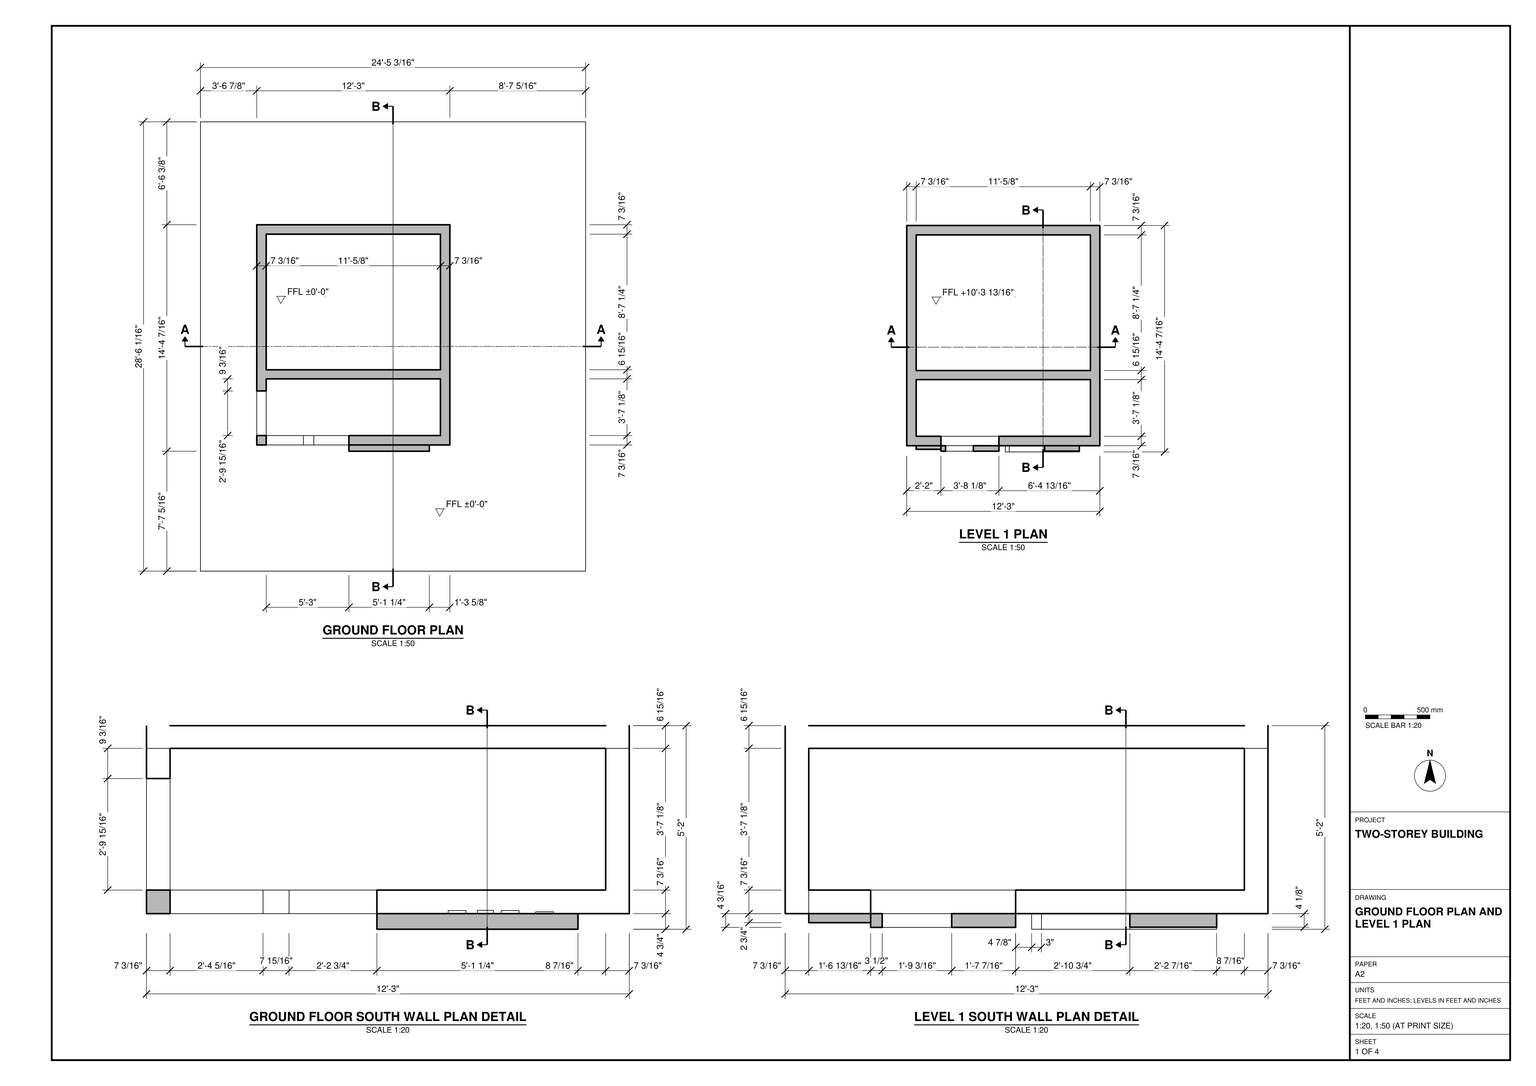
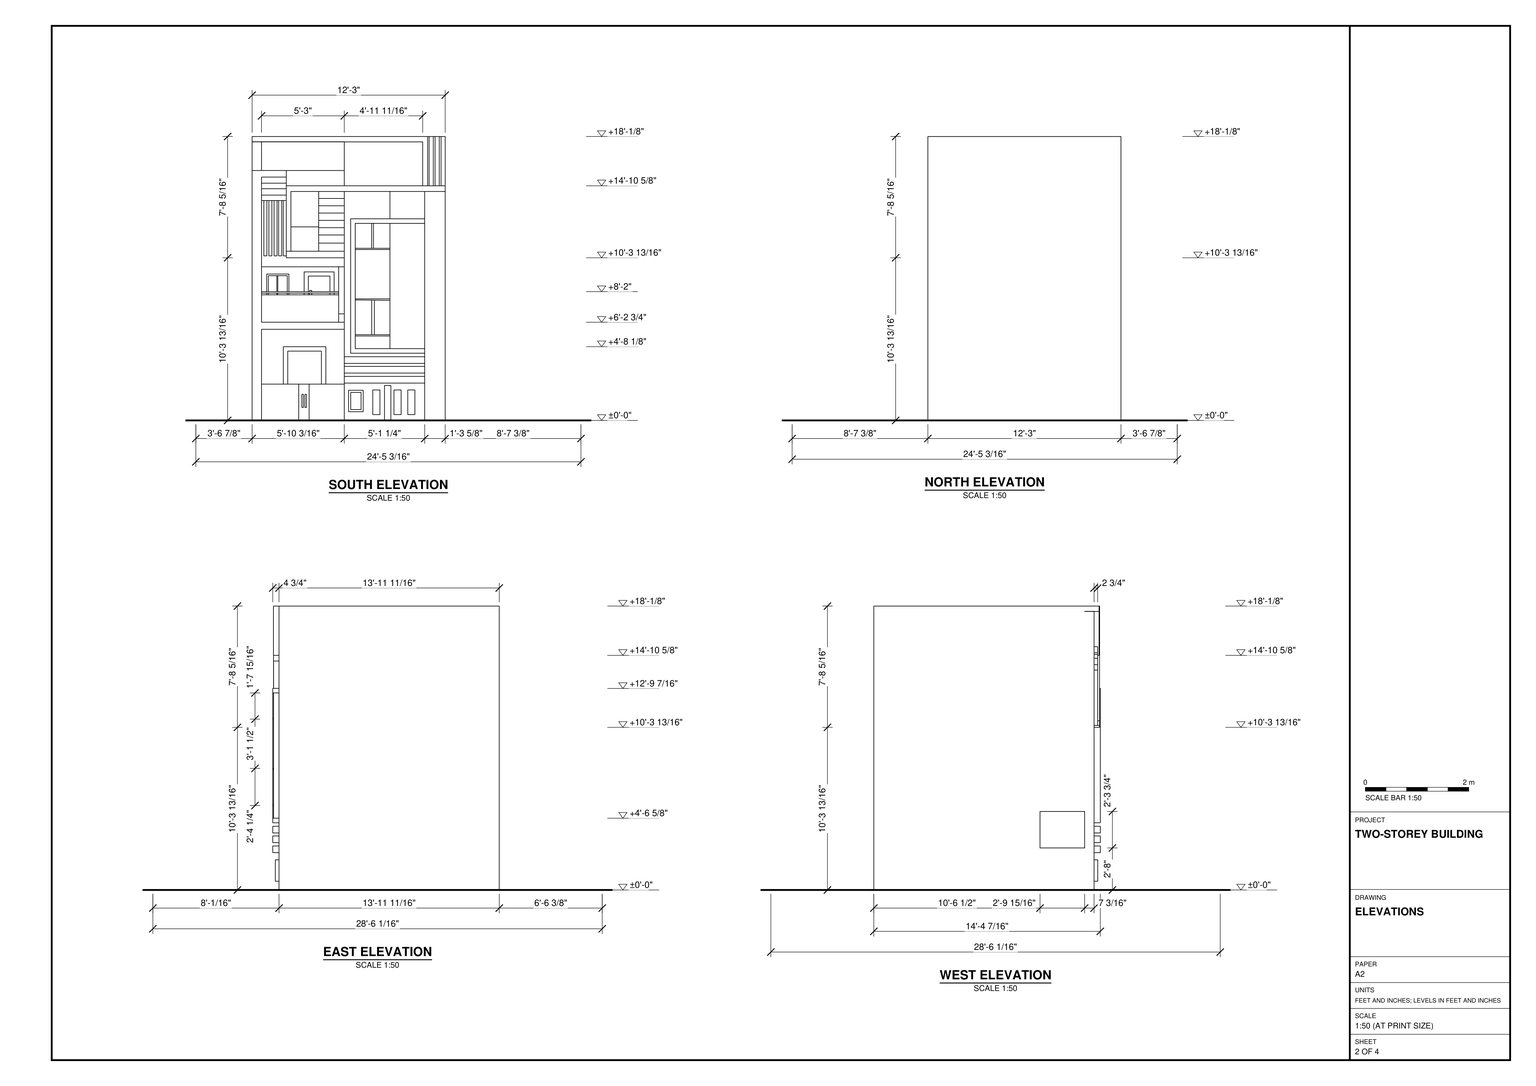
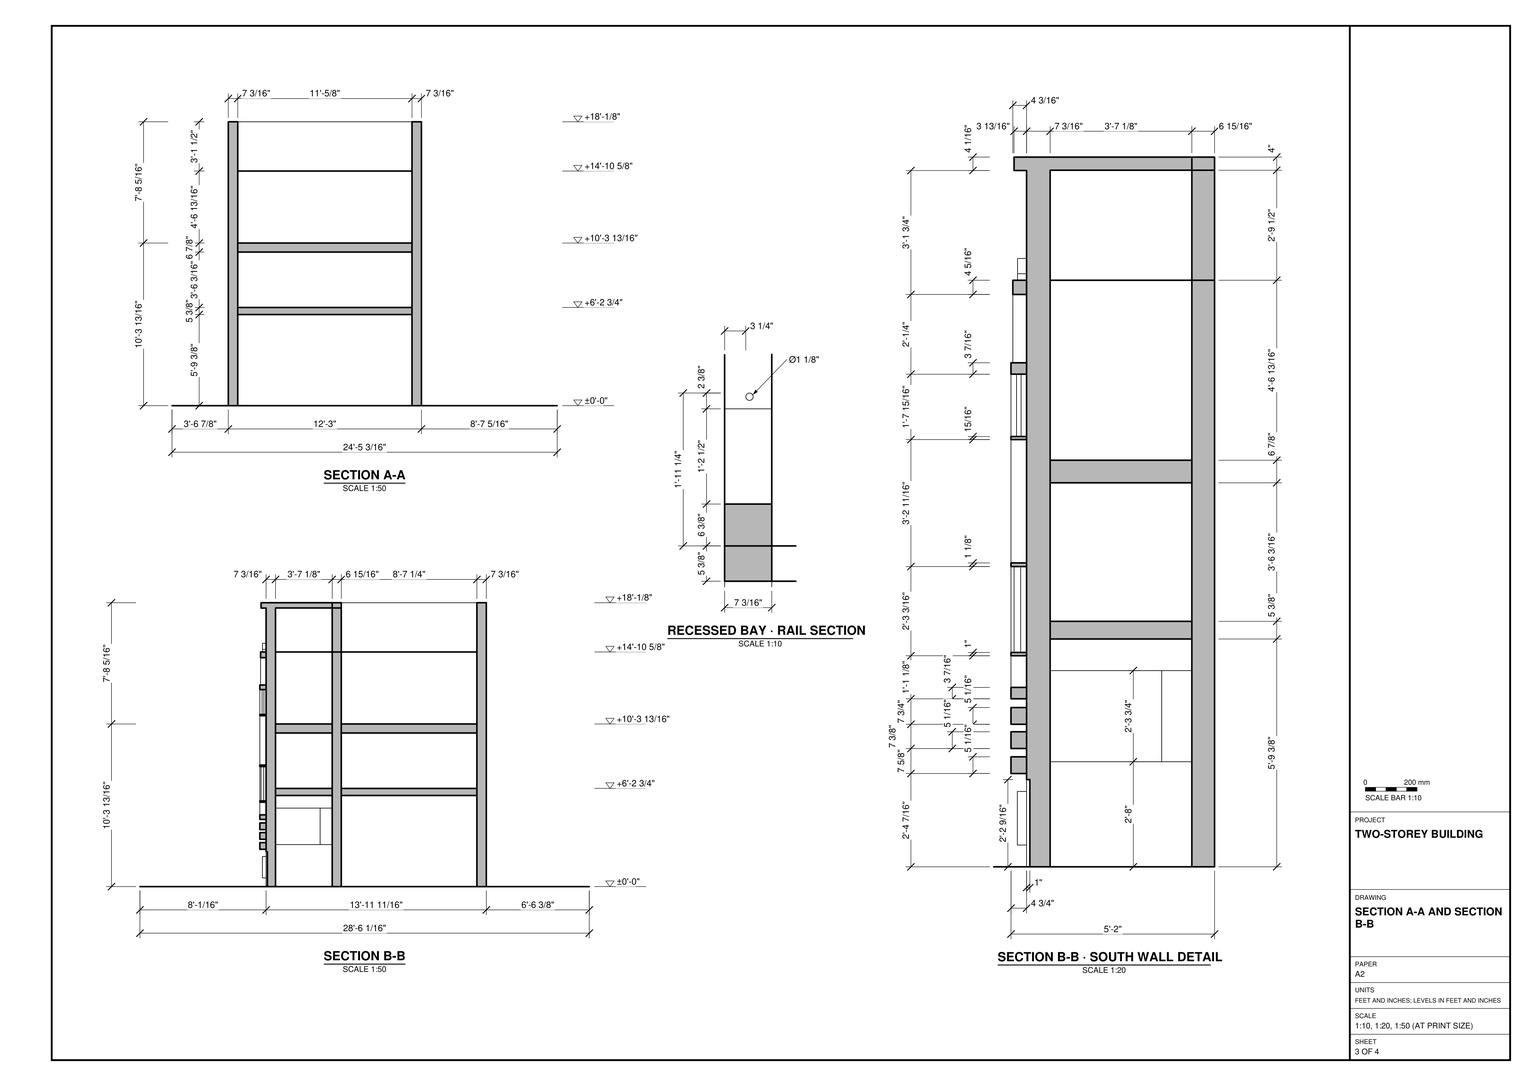
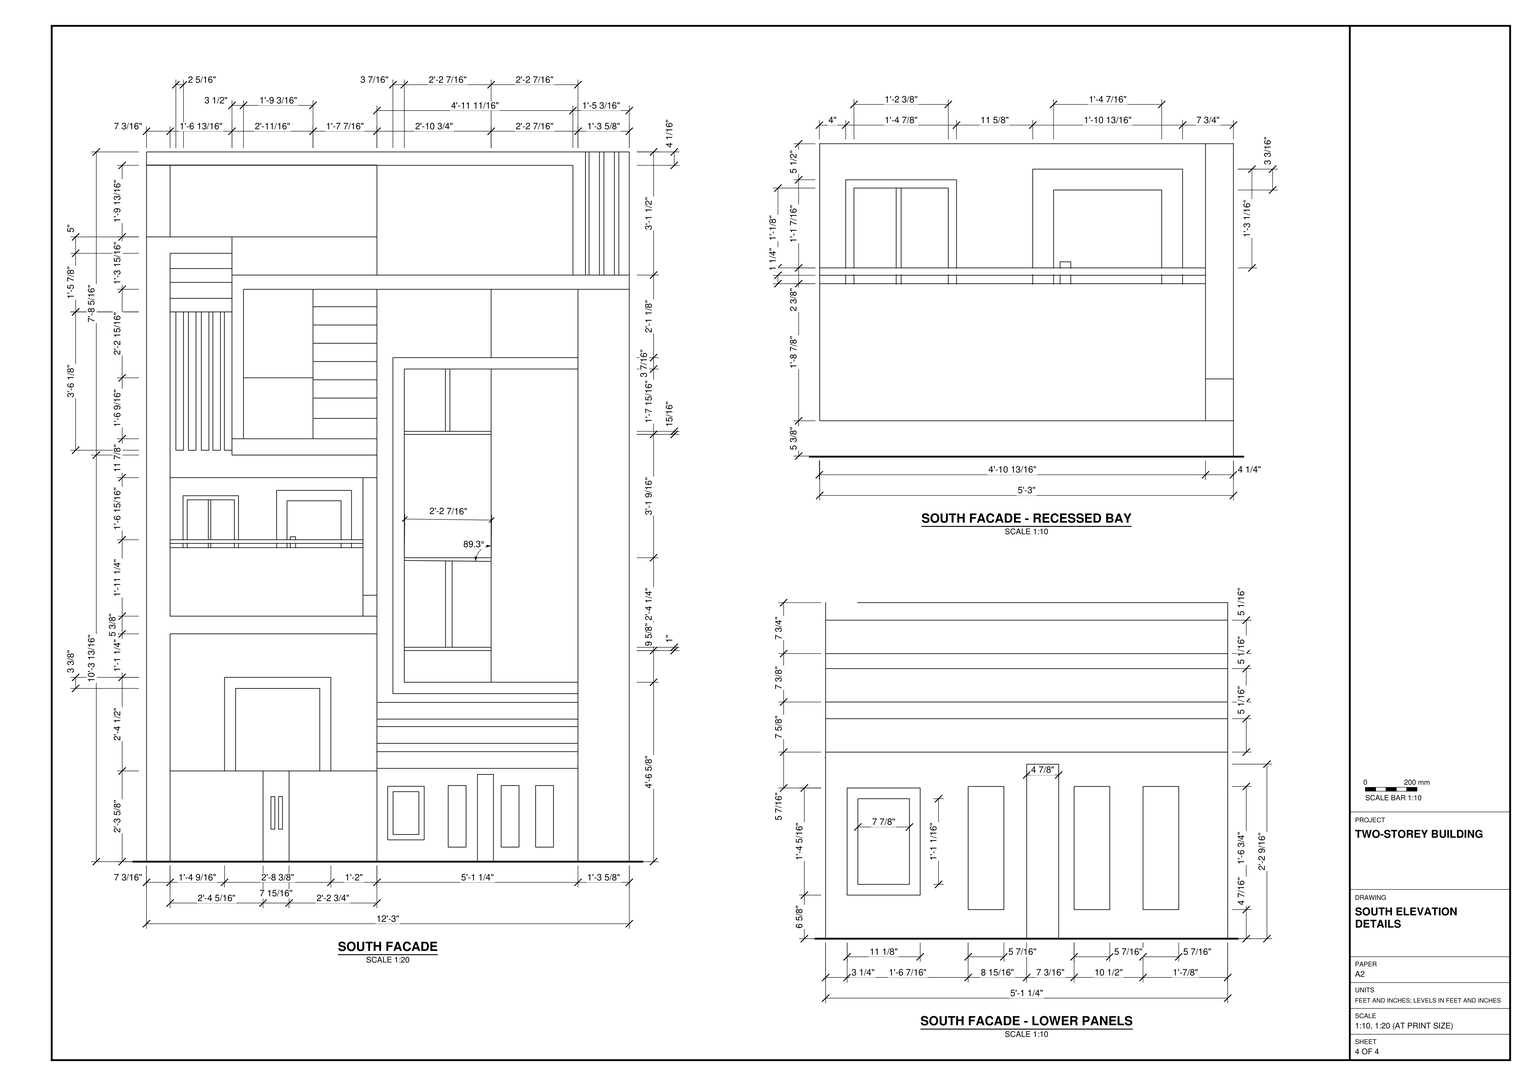
Use task_files/diagram_01.pdf to build the model in SketchUp. Work in feet and inches. Include the rectangular ground plane: the overall model measures 24'-5 3/16" east to west, 28'-6 1/16" north to south and 18'-1/8" high. Set the ground floor at ±0'-0" and Level 1 at +10'-3 13/16". Position the building on the ground plane using the offsets in the ground floor plan rather than centring it.

Build the 12'-3" wide shell with 7 3/16" exterior walls. Set the transverse wall behind the shallow south bay at the thickness shown, leaving the larger space to the north. Use sections A-A and B-B to place the slabs, the intermediate horizontal element below Level 1 and the roof cap over the south bay. Keep the north and east faces plain and include the low opening near the south end of the west wall.

Use the enlarged south wall plans and section to give the frontage depth. Include the entrance panels, recessed bay with its rail, vertical slats, tall framed panel assembly and projecting horizontal bands. Keep shell elements such as walls, slabs and roof, and each furniture or joinery piece, in separate groups or components; use components for repeated parts. Any decor or loose items shown may be suitable library components. Save one SketchUp model as output_files/two_storey_building_with_a_recessed_south_bay.skp.

# SketchUp Ruby script. Lengths in inches.
U = 1.inch
M = Sketchup.active_model
def pt(a) = Geom::Point3d.new(a.map { |v| v * U })
def face(e, loops, mat)
  f = e.add_face(loops[0].map { |a| pt(a) })
  loops[1..].each { |l| e.add_face(l.map { |a| pt(a) }).erase! }
  f.material = f.back_material = mat if mat
  f
end
# faces: each face lists its corners as indices into pts; further lists are holes
def faces(e, pts, list, mat = nil) = list.each { |f| face(e, (f[0].is_a?(Array) ? f : [f]).map { |l| l.map { |i| pts[i] } }, mat) }
# xy, xz, yz: faces in a plane at the given z, y or x. An outline is a flat list of corners, or four numbers for a rectangle; further outlines are holes
def ring(l) = l.size == 4 ? [[l[0], l[1]], [l[2], l[1]], [l[2], l[3]], [l[0], l[3]]] : l.each_slice(2).to_a
def flat(e, list, mat, &to3) = list.each { |f| face(e, (f[0].is_a?(Array) ? f : [f]).map { |l| ring(l).map { |u, v| to3.(u, v) } }, mat) }
def xy(e, z, list, mat = nil) = flat(e, list, mat) { |x, y| [x, y, z] }
def xz(e, y, list, mat = nil) = flat(e, list, mat) { |x, z| [x, y, z] }
def yz(e, x, list, mat = nil) = flat(e, list, mat) { |y, z| [x, y, z] }
def lines(e, pts, list) = list.each { |a, b| e.add_line(pt(pts[a]), pt(pts[b])) }
# prism: a flat outline (further loops are holes) pulled along v
def prism(e, loops, v, mat = nil)
  f = face(e, loops, mat); d = Geom::Vector3d.new(v.map { |x| x * U })
  f.pushpull(f.normal.samedirection?(d) ? d.length : -d.length)
end
def box(e, o, s, mat = nil) = prism(e, [[o, [o[0] + s[0], o[1], o[2]], [o[0] + s[0], o[1] + s[1], o[2]], [o[0], o[1] + s[1], o[2]]]], [0, 0, s[2]], mat)
def at(x, y, z, deg = 0) = Geom::Transformation.translation(pt([x, y, z])) * Geom::Transformation.rotation(ORIGIN, Z_AXIS, deg.degrees)
def axes(o, x, y, z) = Geom::Transformation.new([*x, 0, *y, 0, *z, 0, *pt(o).to_a, 1])
def part(name) = M.definitions.add(name)
# library, detail: a bought-in or finely detailed component or shape, given as its bounding box
def library(name, o, s) = part(name).tap { |d| box(d.entities, o, s) }
def detail(e, o, s) = box(e.add_group.entities, o, s)
def put(e, d, t, mat = nil) = e.add_instance(d, t).tap { |i| i.material = mat if mat }
def group(e, t, mat = nil) = e.add_group.tap { |g| g.transformation = t; g.material = mat if mat }.entities
root = M.entities
M.materials.add("[Aluminum]").color = [179, 179, 179]
M.materials.add("[Asphalt New]").color = [67, 60, 62]
M.materials.add("[Blinds Cellular White]").color = [217, 211, 213]
M.materials.add("[Blinds Cloth Horizontal]").color = [192, 163, 85]
M.materials.add("[Blinds Weave]").color = [141, 91, 25]
M.materials.add("[Color A02]").color = [255, 153, 153]
M.materials.add("[Color A08]").color = [102, 0, 0]
M.materials.add("[Formica Laminate Dark]").color = [50, 53, 60]
M.materials.add("[Formica Laminate Light]").color = [213, 189, 164]
M.materials.add("[Marble Carrara Gold Floor Tile]").color = [225, 223, 217]
M.materials.add("[Polished Concrete Old]").color = [229, 229, 229]
M.materials.add("[Quartz Light Brown]").color = [199, 184, 152]
M.materials.add("[Terrazzo Tile Light]").color = [219, 217, 210]
M.materials.add("[Translucent Glass Blue]").color = [100, 149, 237]
M.materials["[Translucent Glass Blue]"].alpha = 0.5
M.materials.add("[Wood Bamboo]").color = [177, 105, 43]
M.materials.add("[Wood Cherry Original]").color = [152, 86, 42]
M.materials.add("[Wood Floor Dark]").color = [153, 94, 42]
M.materials.add("[Wood OSB]").color = [240, 195, 122]
M.materials.add("[Wood Veneer 01]").color = [120, 70, 37]
M.materials.add("[Wood Veneer 02]").color = [190, 128, 91]
xy(root,0,[[[0,0,293.1875,342.0625],[42.85,96.04,42.85,263.7,189.85,263.7,189.85,96.04,148.5,96.04,148.5,97.04,143.625,97.04,143.625,96.04]],[42.85,96.04,78.34,103.22],[78.34,96.04,86.26,103.22],[86.26,96.04,143.625,96.04,143.625,97.04,148.5,97.04,148.5,96.04,189.85,96.04,189.85,146.37,182.67,146.37,182.67,103.22,86.26,103.22],[42.85,103.22,50.03,146.37],
  [50.03,103.22,182.67,146.37],[[42.85,146.37,189.85,263.7],[50.03,153.28,182.67,256.52]],[50.03,153.28,182.67,256.52]])
xy(root,4.43,[[134.72,96.04,140.15,96.98],[150.84,96.04,156.28,96.98],[161.34,96.04,166.78,96.6]])
xy(root,6.63,[[116.29,93.23,127.41,96.04]])
xy(root,8.27,[[117.92,93.23,125.78,96.04]])
xy(root,21.3125,[[117.92,93.23,125.78,96.04]])
xy(root,22.95,[[116.29,93.23,127.41,96.04]])
xy(root,23.18,[[134.72,96.04,140.15,96.98],[150.84,96.04,156.28,96.98],[161.34,96.04,166.78,96.6]])
xy(root,26.5625,[[143.625,96.04,148.5,97.04]])
xy(root,27.62,[[50.03,96.04,78.34,103.22],[78.34,96.04,86.26,103.22],[86.26,96.04,113.01,103.22]],"[Formica Laminate Dark]")
xy(root,28.41,[[113.01,91.29,174.23,96.04]],"[Color A02]")
xy(root,32,[[42.85,103.22,50.03,137.18]],"[Quartz Light Brown]")
xy(root,33.5,[[113.01,91.29,174.23,96.04]],"[Color A02]")
xy(root,36.03,[[113.01,91.29,174.23,96.04]],"[Color A02]")
xy(root,41.12,[[113.01,91.29,174.23,96.04]],"[Color A02]")
xy(root,43.41,[[113.01,91.29,174.23,96.04]],"[Color A02]")
xy(root,48.5,[[113.01,91.29,174.23,96.04]],"[Color A02]")
xy(root,51.17,[[117.88,91.29,120.88,96.04],[120.88,91.29,174.23,96.04]])
xy(root,54.64,[[147.79,91.29,174.23,91.91],[147.79,91.91,174.23,96.04]])
xy(root,54.64,[[121.35,91.29,147.79,96.04]],"[Wood Veneer 01]")
xy(root,59.75,[[42.85,103.22,50.03,137.18]])
xy(root,64.28,[[121.35,91.29,147.79,96.04]],"[Wood Veneer 01]")
xy(root,65.28,[[[121.35,91.29,147.79,96.04],[134.91,92.23,134.65,92.26,134.41,92.36,134.2,92.52,134.05,92.73,133.95,92.97,133.91,93.23,133.95,93.49,134.05,93.73,134.2,93.9375,134.41,94.1,134.65,94.2,134.91,94.23,135.17,94.2,135.41,94.1,135.62,93.9375,135.78,93.73,135.88,93.49,135.91,93.23,135.88,92.97,135.78,92.73,135.62,92.52,135.41,92.36,135.17,92.26]],[134.91,92.23,134.65,92.26,134.41,92.36,134.2,92.52,134.05,92.73,133.95,92.97,133.91,93.23,133.95,93.49,134.05,93.73,134.2,93.9375,134.41,94.1,134.65,94.2,134.91,94.23,135.17,94.2,135.41,94.1,135.62,93.9375,135.78,93.73,135.88,93.49,135.91,93.23,135.88,92.97,135.78,92.73,135.62,92.52,135.41,92.36,135.17,92.26]])
xy(root,69.375,[[50.03,96.04,113.01,103.22],[50.03,103.22,182.67,146.37],[50.03,153.28,182.67,256.52]])
xy(root,74.75,[[50.03,96.04,113.01,103.22],[50.03,103.22,182.67,146.37],[50.03,153.28,182.67,256.52]])
xy(root,81.125,[[108.76,96.04,113.01,103.22]])
xy(root,91.5625,[[134.91,92.23,135.17,92.26,135.41,92.36,135.62,92.52,135.78,92.73,135.88,92.97,135.91,93.23,135.88,93.49,135.78,93.73,135.62,93.9375,135.41,94.1,135.17,94.2,134.91,94.23,134.65,94.2,134.41,94.1,134.2,93.9375,134.05,93.73,133.95,93.49,133.91,93.23,133.95,92.97,134.05,92.73,134.2,92.52,134.41,92.36,134.65,92.26]])
xy(root,92.55,[[121.35,91.29,147.79,96.04]],"[Wood Veneer 01]")
xy(root,95.625,[[50.03,96.04,108.76,103.22]],"[Translucent Glass Blue]")
xy(root,116.9375,[[50.03,96.04,108.76,103.22],[108.76,96.04,113.01,103.22],[50.03,103.22,182.67,146.37],[50.03,153.28,182.67,256.52]])
xy(root,123.8125,[[68.87,96.04,113.01,103.22],[50.03,103.22,182.67,146.37],[50.03,153.28,182.67,256.52]])
xy(root,123.8125,[[68.87,91.85,113.01,96.04]],"[Color A08]")
xy(root,125.28,[[51.8,93.29,54.11,96.04],[55.61,93.29,57.92,96.04],[59.55,93.29,61.86,96.04],[63.05,93.29,65.37,96.04],[66.56,93.29,68.87,96.04]])
xy(root,128.78,[[68.87,91.85,72.38,96.04]])
xy(root,128.78,[[72.38,91.85,93.55,96.04]],"[Color A08]")
xy(root,130.1,[[121.35,91.29,147.79,96.04]],"[Wood Veneer 01]")
xy(root,131.04,[[[121.35,91.29,147.79,96.04],[134.55,92.99,134.37,93.01,134.2,93.08,134.0625,93.19,133.95,93.33,133.88,93.5,133.86,93.68,133.88,93.85,133.95,94.02,134.0625,94.16,134.2,94.27,134.37,94.34,134.55,94.36,134.73,94.34,134.89,94.27,135.03,94.16,135.14,94.02,135.21,93.85,135.24,93.68,135.21,93.5,135.14,93.33,135.03,93.19,134.89,93.08,134.73,93.01]],[134.55,92.99,134.37,93.01,134.2,93.08,134.0625,93.19,133.95,93.33,133.88,93.5,133.86,93.68,133.88,93.85,133.95,94.02,134.0625,94.16,134.2,94.27,134.37,94.34,134.55,94.36,134.73,94.34,134.89,94.27,135.03,94.16,135.14,94.02,135.21,93.85,135.24,93.68,135.21,93.5,135.14,93.33,135.03,93.19,134.89,93.08,134.73,93.01]])
xy(root,147.34,[[68.87,96.04,113.01,103.22]],"[Translucent Glass Blue]")
xy(root,150.02,[[[121.35,91.29,147.79,96.04],[134.55,92.99,134.73,93.01,134.89,93.08,135.03,93.19,135.14,93.33,135.21,93.5,135.24,93.68,135.21,93.85,135.14,94.02,135.03,94.16,134.89,94.27,134.73,94.34,134.55,94.36,134.37,94.34,134.2,94.27,134.0625,94.16,133.95,94.02,133.88,93.85,133.86,93.68,133.88,93.5,133.95,93.33,134.0625,93.19,134.2,93.08,134.37,93.01]],[147.79,91.29,174.23,91.91],[147.79,91.91,174.23,96.04]])
xy(root,153.49,[[117.88,91.29,120.88,96.04],[120.88,91.29,147.79,96.04],[147.79,91.29,174.23,91.91],[147.79,91.91,174.23,96.04]])
xy(root,167.41,[[50.03,93.29,51.8,96.04],[51.8,93.29,54.11,96.04],[54.11,93.29,55.61,96.04],[55.61,93.29,57.92,96.04],[57.92,93.29,59.55,96.04],
  [59.55,93.29,61.86,96.04],[61.86,93.29,63.05,96.04],[63.05,93.29,65.37,96.04],[65.37,93.29,66.56,96.04],[66.56,93.29,68.87,96.04]])
xy(root,171.54,[[50.03,93.29,68.87,96.04]])
xy(root,174.29,[[147.79,91.91,174.23,96.04],[68.87,96.04,113.01,103.22]])
xy(root,174.29,[[72.38,91.85,93.55,96.04],[113.01,91.85,113.01,96.04,147.79,96.04,147.79,91.91,174.23,91.91,174.23,96.04,189.85,96.04,189.85,91.85]],"[Color A08]")
xy(root,176.39,[[50.03,93.29,68.87,96.04]])
xy(root,178.625,[[172.7,92.23,176.51,96.04],[68.87,96.04,113.01,103.22],[50.03,103.22,182.67,146.37],[50.03,146.37,114.88,153.28],[114.88,146.37,182.67,153.28],
  [50.03,153.28,182.67,256.52]])
xy(root,178.625,[[177.6,91.79,180.78,91.85],[182.14,91.79,185.32,91.85],[186.67,91.79,189.85,91.85],[68.87,91.85,177.6,91.85,177.6,96.04,176.51,96.04,176.51,92.23,172.7,92.23,172.7,96.04,68.87,96.04],[177.6,91.85,180.78,96.04],
  [180.78,91.85,182.14,96.04],[182.14,91.85,185.32,96.04],[185.32,91.85,186.67,96.04],[186.67,91.85,189.85,96.04]],"[Color A08]")
xy(root,180.62,[[50.03,93.29,68.87,96.04]])
xy(root,185.26,[[50.03,93.29,68.87,96.04]],"[Wood Cherry Original]")
xy(root,190.25,[[50.03,96.04,68.87,103.22]],"[Color A08]")
xy(root,190.25,[[68.87,96.04,113.01,103.22]],"[Translucent Glass Blue]")
xy(root,212.04,[[113.01,92.23,172.7,96.04],[42.85,96.04,50.03,103.22]])
xy(root,212.04,[[42.85,92.23,50.03,95.84],[50.03,92.23,113.01,96.04],[42.85,95.84,50.03,96.04]],"[Color A08]")
xy(root,212.125,[[42.85,95.84,50.03,103.22],[114.88,146.37,182.67,153.28]])
xy(root,212.125,[[[50.03,103.22,182.67,146.37],[55.6875,107.83,60.6875,139.15],[62.5,107.83,67.5,139.15],[69.5,107.83,74.5,139.15],[76.75,107.83,81.75,139.15],[84.0625,107.83,89.0625,139.15],[91.625,107.83,96.625,139.15],[99.5625,107.83,104.5625,139.15],[106.9375,107.83,111.9375,139.15]]],"[Quartz Light Brown]")
xy(root,216.125,[[[50.03,103.22,182.67,146.37],[55.6875,107.83,60.6875,139.15],[62.5,107.83,67.5,139.15],[69.5,107.83,74.5,139.15],[76.75,107.83,81.75,139.15],[84.0625,107.83,89.0625,139.15],[91.625,107.83,96.625,139.15],[99.5625,107.83,104.5625,139.15],[106.9375,107.83,111.9375,139.15]]],"[Color A08]")
xy(root,216.125,[[177.6,91.79,180.78,96.04],[182.14,91.79,185.32,96.04],[186.67,91.79,189.85,96.04]],"[Polished Concrete Old]")
xy(root,216.125,[[42.85,92.23,176.51,92.23,176.51,96.04,189.85,96.04,189.85,263.7,42.85,263.7,42.85,103.22,50.03,103.22,50.03,256.52,182.67,256.52,182.67,153.28,114.88,153.28,114.88,146.37,182.67,146.37,182.67,103.22,42.85,103.22]],"[Quartz Light Brown]")
xz(root,91.29,[[117.88,51.17,174.23,51.17,174.23,54.64,121.35,54.64,121.35,150.02,174.23,150.02,174.23,153.49,117.88,153.49],[121.35,64.28,147.79,65.28],[147.79,91.42,147.79,92.55,121.35,92.55,121.35,91.74],[121.35,130.1,147.79,131.04]])
xz(root,91.29,[[113.01,28.41,174.23,33.5],[113.01,36.03,174.23,41.12],[113.01,43.41,174.23,48.5]],"[Color A02]")
xz(root,91.79,[[177.6,178.625,180.78,216.125],[182.14,178.625,185.32,216.125],[186.67,178.625,189.85,216.125]],"[Polished Concrete Old]")
xz(root,91.85,[[68.87,123.8125,113.01,128.78],[68.87,128.78,72.38,128.78,72.38,174.29,189.85,174.29,189.85,178.625,68.87,178.625]],"[Color A08]")
xz(root,91.85,[[93.55,128.78,113.01,134.98],[93.55,134.98,113.01,141.17],[93.55,141.17,113.01,146.73],[93.55,146.73,113.01,152.3],[93.55,152.3,113.01,157.86],
  [93.55,157.86,113.01,163.42],[93.55,163.42,113.01,168.98],[93.55,168.98,113.01,174.29]],"[Wood Bamboo]")
xz(root,91.91,[[147.79,54.64,174.23,150.02],[147.79,153.49,174.23,174.29]],"[Marble Carrara Gold Floor Tile]")
xz(root,92.23,[[172.7,178.625,176.51,178.625,176.51,216.125,42.85,216.125,42.85,212.04,172.7,212.04]],"[Color A08]")
xz(root,93.23,[[[116.29,6.63,127.41,22.95],[117.92,8.27,125.78,21.3125]]],"[Asphalt New]")
xz(root,93.29,[[51.8,125.28,54.11,167.41],[55.61,125.28,57.92,167.41],[59.55,125.28,61.86,167.41],[63.05,125.28,65.37,167.41],[66.56,125.28,68.87,167.41]],"[Formica Laminate Dark]")
xz(root,93.29,[[50.03,167.41,68.87,171.54],[50.03,171.54,68.87,176.39],[50.03,176.39,68.87,180.62],[50.03,180.62,68.87,185.26]],"[Wood Cherry Original]")
xz(root,95.84,[[42.85,212.04,50.03,212.125]])
xz(root,96.04,[[[116.29,6.63,127.41,22.95],[117.92,8.27,125.78,21.3125]],[80.74,9.89,81.93,19.83],[83.06,9.89,84.24,19.83],[113.01,28.41,174.23,33.5],[113.01,33.5,174.23,36.03],
  [113.01,36.03,174.23,41.12],[113.01,41.12,174.23,43.41],[113.01,43.41,174.23,48.5],[117.88,51.17,117.88,153.49,147.79,153.49,147.79,150.02,121.35,150.02,121.35,54.64,174.23,54.64,174.23,51.17],[147.79,54.64,174.23,150.02],
  [121.35,64.28,147.79,65.28],[147.79,91.42,121.35,91.74,121.35,92.55,147.79,92.55],[68.87,123.8125,68.87,128.78,93.55,128.78,93.55,147.34,113.01,147.34,113.01,123.8125],[51.8,125.28,54.11,167.41],[55.61,125.28,57.92,167.41],
  [59.55,125.28,61.86,167.41],[63.05,125.28,65.37,167.41],[66.56,125.28,68.87,167.41],[68.87,128.78,72.38,147.34],[121.35,130.1,147.79,131.04],
  [68.87,147.34,72.38,174.29],[93.55,147.34,113.01,174.29],[147.79,150.02,174.23,153.49],[147.79,153.49,174.23,174.29],[50.03,167.41,68.87,171.54],
  [50.03,171.54,68.87,176.39],[68.87,174.29,113.01,178.625],[113.01,174.29,189.85,178.625],[50.03,176.39,68.87,180.62],[50.03,180.62,68.87,185.26]])
xz(root,96.04,[[117.92,8.27,125.78,21.3125]],"[Asphalt New]")
xz(root,96.04,[[121.35,65.28,147.79,65.28,147.79,91.42,121.35,91.74],[121.35,131.04,147.79,150.02]],"[Blinds Cellular White]")
xz(root,96.04,[[113.01,178.625,172.7,212.04]],"[Blinds Weave]")
xz(root,96.04,[[42.85,0,50.03,0,50.03,69.375,113.01,69.375,113.01,74.75,50.03,74.75,50.03,185.26,68.87,185.26,68.87,190.25,42.85,190.25],[174.23,0,189.85,174.29],[113.01,48.5,174.23,48.5,174.23,51.17,117.88,51.17,117.88,153.49,147.79,153.49,147.79,174.29,113.01,174.29],[177.6,178.625,180.78,216.125],[182.14,178.625,185.32,216.125],
  [186.67,178.625,189.85,216.125],[42.85,190.25,50.03,212.04]],"[Color A08]")
xz(root,96.04,[[50.03,0,78.34,27.62],[[78.34,0,86.26,27.62],[80.74,9.89,81.93,19.83],[83.06,9.89,84.24,19.83]],[86.26,0,113.01,27.62]],"[Formica Laminate Dark]")
xz(root,96.04,[[176.51,178.625,177.6,216.125],[180.78,178.625,182.14,216.125],[185.32,178.625,186.67,216.125]],"[Polished Concrete Old]")
xz(root,96.04,[[[113.01,0,143.625,0,143.625,26.5625,148.5,26.5625,148.5,0,174.23,0,174.23,28.41,113.01,28.41],[116.29,6.63,127.41,22.95],[134.72,4.43,140.15,23.18],[150.84,4.43,156.28,23.18],[161.34,4.43,166.78,23.18]],[108.76,74.75,113.01,81.125],[108.76,81.125,113.01,116.9375],[50.03,116.9375,113.01,116.9375,113.01,123.8125,68.87,123.8125,68.87,125.28,66.56,125.28,66.56,167.41,65.37,167.41,65.37,125.28,63.05,125.28,63.05,167.41,61.86,167.41,61.86,125.28,59.55,125.28,59.55,167.41,57.92,167.41,57.92,125.28,55.61,125.28,55.61,167.41,54.11,167.41,54.11,125.28,51.8,125.28,51.8,167.41,50.03,167.41]],"[Quartz Light Brown]")
xz(root,96.04,[[50.03,74.75,108.76,95.625],[72.38,128.78,93.55,147.34],[68.87,178.625,113.01,190.25]],"[Translucent Glass Blue]")
xz(root,96.04,[[121.35,54.64,147.79,64.28],[121.35,92.55,147.79,130.1]],"[Wood Veneer 01]")
xz(root,96.6,[[161.34,4.43,166.78,23.18]],"[Terrazzo Tile Light]")
xz(root,96.98,[[134.72,4.43,140.15,23.18],[150.84,4.43,156.28,23.18]],"[Terrazzo Tile Light]")
xz(root,97.04,[[143.625,0,148.5,26.5625]],"[Terrazzo Tile Light]")
xz(root,103.22,[[50.03,0,78.34,27.62],[78.34,0,86.26,27.62],[50.03,69.375,113.01,74.75],[113.01,69.375,182.67,74.75],[50.03,74.75,50.03,95.625,108.76,95.625,108.76,81.125,113.01,81.125,113.01,74.75],
  [113.01,74.75,113.01,81.125,108.76,81.125,108.76,116.9375,182.67,116.9375,182.67,74.75],[50.03,116.9375,113.01,123.8125],[113.01,116.9375,182.67,123.8125],[50.03,123.8125,68.87,178.625],[68.87,123.8125,68.87,147.34,113.01,147.34,113.01,178.625,182.67,178.625,182.67,123.8125],
  [68.87,174.29,113.01,178.625],[42.85,212.04,50.03,212.125]])
xz(root,103.22,[[86.26,0,86.26,27.62,113.01,27.62,113.01,69.375,182.67,69.375,182.67,0],[42.85,32,50.03,59.75],[50.03,178.625,68.87,190.25],[68.87,178.625,113.01,190.25],[113.01,178.625,182.67,212.125]],"[Quartz Light Brown]")
xz(root,107.83,[[55.6875,212.125,60.6875,216.125],[62.5,212.125,67.5,216.125],[69.5,212.125,74.5,216.125],[76.75,212.125,81.75,216.125],[84.0625,212.125,89.0625,216.125],
  [91.625,212.125,96.625,216.125],[99.5625,212.125,104.5625,216.125],[106.9375,212.125,111.9375,216.125]])
xz(root,137.18,[[42.85,32,50.03,59.75]],"[Quartz Light Brown]")
xz(root,139.15,[[55.6875,212.125,60.6875,216.125],[62.5,212.125,67.5,216.125],[69.5,212.125,74.5,216.125],[76.75,212.125,81.75,216.125],[84.0625,212.125,89.0625,216.125],
  [91.625,212.125,96.625,216.125],[99.5625,212.125,104.5625,216.125],[106.9375,212.125,111.9375,216.125]])
xz(root,146.37,[[50.03,69.375,182.67,74.75],[86.63,90.51,88.25,98.95],[50.03,116.9375,182.67,123.8125],[114.88,212.125,182.67,216.125]])
xz(root,146.37,[[55.24,89.07,61.67,110.18],[62.42,89.07,69.6,110.18]],"[Blinds Cloth Horizontal]")
xz(root,146.37,[[[50.03,74.75,82.46,74.75,82.46,113.0625,105.27,113.0625,105.27,74.75,182.67,74.75,182.67,116.9375,50.03,116.9375],[53.98,87.82,70.86,111.44]]],"[Formica Laminate Light]")
xz(root,146.37,[[50.03,0,66.61,0,66.61,56.125,98.99,56.125,98.99,0,182.67,0,182.67,69.375,50.03,69.375],[114.88,178.625,182.67,212.125],[50.03,212.125,114.88,216.125]],"[Quartz Light Brown]")
xz(root,146.37,[[[82.46,74.75,105.27,113.0625],[85.64,77.92,102.1,109.89]],[[85.64,77.92,102.1,109.89],[86.63,90.51,88.25,98.95]]],"[Wood Floor Dark]")
xz(root,146.37,[[50.03,123.8125,182.67,178.625]],"[Wood OSB]")
xz(root,146.37,[[[66.61,0,98.99,56.125],[69.99,3.375,95.61,52.75]],[69.99,3.375,95.61,52.75]],"[Wood Veneer 01]")
xz(root,146.37,[[[53.98,87.82,70.86,111.44],[55.24,89.07,69.6,110.18]],[61.67,89.07,62.42,110.18]],"[Wood Veneer 02]")
xz(root,153.28,[[50.03,0,182.67,69.375],[50.03,69.375,182.67,74.75],[50.03,74.75,182.67,116.9375],[50.03,116.9375,182.67,123.8125],[50.03,123.8125,182.67,178.625]])
xz(root,153.28,[[114.88,178.625,182.67,212.125],[114.88,212.125,182.67,216.125]],"[Quartz Light Brown]")
xz(root,256.52,[[50.03,0,182.67,69.375],[50.03,69.375,182.67,74.75],[50.03,74.75,182.67,116.9375],[50.03,116.9375,182.67,123.8125],[50.03,123.8125,182.67,178.625]])
xz(root,256.52,[[50.03,178.625,182.67,216.125]],"[Quartz Light Brown]")
xz(root,263.7,[[42.85,0,189.85,216.125]],"[Quartz Light Brown]")
yz(root,42.85,[[[96.04,0,96.04,212.04,103.22,212.04,103.22,212.125,95.84,212.125,95.84,212.04,92.23,212.04,92.23,216.125,263.7,216.125,263.7,0],[103.22,32,137.18,59.75]],[95.84,212.04,95.84,212.125,103.22,212.125,96.04,212.04],[96.04,212.04,103.22,212.125,103.22,212.04]],"[Quartz Light Brown]")
yz(root,49.76,[[99.82,96.91,99.68,96.93,99.54,96.98,99.43,97.07,99.34,97.1875,99.28,97.32,99.26,97.47,99.28,97.61,99.34,97.75,99.43,97.87,99.54,97.96,99.68,98.01,99.82,98.03,99.97,98.01,100.11,97.96,100.22,97.87,100.3125,97.75,100.37,97.61,100.39,97.47,100.37,97.32,100.3125,97.1875,100.22,97.07,100.11,96.98,99.97,96.93]])
yz(root,50.03,[[153.28,0,256.52,69.375],[103.22,69.375,146.37,74.75],[153.28,69.375,256.52,74.75],[96.04,74.75,103.22,95.625],[153.28,74.75,256.52,116.9375],
  [96.04,116.9375,103.22,123.8125],[103.22,116.9375,146.37,123.8125],[153.28,116.9375,256.52,123.8125],[153.28,123.8125,256.52,178.625],[95.84,212.04,103.22,212.125]])
yz(root,50.03,[[96.04,190.25,103.22,212.04]],"[Color A08]")
yz(root,50.03,[[103.22,74.75,146.37,116.9375],[96.04,95.625,103.22,116.9375]],"[Formica Laminate Light]")
yz(root,50.03,[[103.22,0,146.37,32],[96.04,27.62,103.22,69.375],[137.18,32,146.37,59.75],[103.22,59.75,146.37,69.375],[103.22,178.625,153.28,178.625,153.28,216.125,146.37,216.125,146.37,212.125,103.22,212.125],
  [153.28,178.625,256.52,216.125]],"[Quartz Light Brown]")
yz(root,50.03,[[93.29,167.41,96.04,171.54],[93.29,171.54,96.04,176.39],[93.29,176.39,96.04,179.3125],[93.29,179.3125,96.04,180.62],[93.29,180.62,96.04,185.26]],"[Wood Cherry Original]")
yz(root,50.03,[[103.22,123.8125,146.37,178.625]],"[Wood OSB]")
yz(root,51.8,[[93.29,125.28,96.04,167.41]],"[Formica Laminate Dark]")
yz(root,54.11,[[93.29,125.28,96.04,167.41]],"[Formica Laminate Dark]")
yz(root,55.61,[[93.29,125.28,96.04,167.41]],"[Formica Laminate Dark]")
yz(root,55.6875,[[107.83,212.125,139.15,216.125]])
yz(root,57.92,[[93.29,125.28,96.04,167.41]],"[Formica Laminate Dark]")
yz(root,59.55,[[93.29,125.28,96.04,167.41]],"[Formica Laminate Dark]")
yz(root,60.6875,[[107.83,212.125,139.15,216.125]])
yz(root,61.86,[[93.29,125.28,96.04,167.41]],"[Formica Laminate Dark]")
yz(root,62.5,[[107.83,212.125,139.15,216.125]])
yz(root,63.05,[[93.29,125.28,96.04,167.41]],"[Formica Laminate Dark]")
yz(root,65.37,[[93.29,125.28,96.04,167.41]],"[Formica Laminate Dark]")
yz(root,66.56,[[93.29,125.28,96.04,167.41]],"[Formica Laminate Dark]")
yz(root,67.5,[[107.83,212.125,139.15,216.125]])
yz(root,68.87,[[93.29,125.28,96.04,128.78],[93.29,128.78,96.04,167.41],[96.04,147.34,103.22,174.29],[93.29,167.41,96.04,171.54],[93.29,171.54,96.04,176.39],
  [96.04,174.29,103.22,178.625],[93.29,176.39,96.04,178.625],[96.04,178.625,103.22,190.25]])
yz(root,68.87,[[91.85,123.8125,96.04,125.28],[91.85,125.28,93.29,128.78],[91.85,128.78,93.29,178.625]],"[Color A08]")
yz(root,68.87,[[93.29,178.625,96.04,180.62],[93.29,180.62,96.04,185.26]],"[Wood Cherry Original]")
yz(root,69.5,[[107.83,212.125,139.15,216.125]])
yz(root,72.38,[[91.85,128.78,96.04,174.29]],"[Color A08]")
yz(root,74.5,[[107.83,212.125,139.15,216.125]])
yz(root,76.75,[[107.83,212.125,139.15,216.125]])
yz(root,78.34,[[96.04,0,103.22,27.62]])
yz(root,81.75,[[107.83,212.125,139.15,216.125]])
yz(root,84.0625,[[107.83,212.125,139.15,216.125]])
yz(root,86.26,[[96.04,0,103.22,27.62]])
yz(root,89.0625,[[107.83,212.125,139.15,216.125]])
yz(root,91.625,[[107.83,212.125,139.15,216.125]])
yz(root,93.55,[[91.85,128.78,96.04,174.29]],"[Wood Bamboo]")
yz(root,96.625,[[107.83,212.125,139.15,216.125]])
yz(root,99.5625,[[107.83,212.125,139.15,216.125]])
yz(root,104.5625,[[107.83,212.125,139.15,216.125]])
yz(root,106.9375,[[107.83,212.125,139.15,216.125]])
yz(root,108.76,[[96.04,81.125,103.22,95.625],[99.82,96.91,99.97,96.93,100.11,96.98,100.22,97.07,100.3125,97.1875,100.37,97.32,100.39,97.47,100.37,97.61,100.3125,97.75,100.22,97.87,100.11,97.96,99.97,98.01,99.82,98.03,99.68,98.01,99.54,97.96,99.43,97.87,99.34,97.75,99.28,97.61,99.26,97.47,99.28,97.32,99.34,97.1875,99.43,97.07,99.54,96.98,99.68,96.93]])
yz(root,108.76,[[[96.04,95.625,103.22,116.9375],[99.82,96.91,99.97,96.93,100.11,96.98,100.22,97.07,100.3125,97.1875,100.37,97.32,100.39,97.47,100.37,97.61,100.3125,97.75,100.22,97.87,100.11,97.96,99.97,98.01,99.82,98.03,99.68,98.01,99.54,97.96,99.43,97.87,99.34,97.75,99.28,97.61,99.26,97.47,99.28,97.32,99.34,97.1875,99.43,97.07,99.54,96.98,99.68,96.93]]],"[Quartz Light Brown]")
yz(root,111.9375,[[107.83,212.125,139.15,216.125]])
yz(root,113.01,[[96.04,69.375,103.22,74.75],[96.04,74.75,103.22,81.125],[96.04,116.9375,103.22,123.8125],[96.04,147.34,103.22,174.29],[96.04,174.29,103.22,178.625]])
yz(root,113.01,[[96.04,190.25,96.04,212.04,103.22,212.125,103.22,190.25]],"[Blinds Weave]")
yz(root,113.01,[[91.29,28.41,96.04,33.5],[91.29,36.03,96.04,41.12],[91.29,43.41,96.04,48.5]],"[Color A02]")
yz(root,113.01,[[91.85,123.8125,96.04,174.29]],"[Color A08]")
yz(root,113.01,[[96.04,27.62,103.22,69.375]],"[Quartz Light Brown]")
yz(root,114.88,[[146.37,178.625,153.28,212.125],[146.37,212.125,153.28,216.125]],"[Quartz Light Brown]")
yz(root,116.29,[[93.23,6.63,96.04,22.95]])
yz(root,117.88,[[91.29,51.17,96.04,153.49]])
yz(root,117.92,[[93.23,8.27,96.04,21.3125]],"[Asphalt New]")
yz(root,121.35,[[91.29,64.28,96.04,65.28],[91.29,65.28,96.04,91.74],[91.29,91.74,96.04,92.55],[91.29,130.1,96.04,131.04],[91.29,131.04,96.04,150.02]])
yz(root,121.35,[[91.29,54.64,96.04,64.28],[91.29,92.55,96.04,130.1]],"[Wood Veneer 01]")
yz(root,125.78,[[93.23,8.27,96.04,21.3125]],"[Asphalt New]")
yz(root,127.41,[[93.23,6.63,96.04,22.95]])
yz(root,134.72,[[96.04,4.43,96.98,23.18]])
yz(root,140.15,[[96.04,4.43,96.98,23.18]])
yz(root,143.625,[[96.04,0,97.04,26.5625]])
yz(root,147.79,[[91.29,64.28,91.91,65.28],[91.91,64.28,96.04,65.28],[91.29,91.42,91.91,92.17],[91.91,91.42,96.04,92.17],[91.29,92.17,91.91,92.55],
  [91.91,92.17,96.04,92.55],[91.29,130.1,91.91,131.04],[91.91,130.1,96.04,131.04]])
yz(root,147.79,[[91.91,65.28,96.04,91.42],[91.91,131.04,96.04,150.02],[91.91,153.49,96.04,174.29]],"[Marble Carrara Gold Floor Tile]")
yz(root,147.79,[[91.91,54.64,96.04,64.28],[91.91,92.55,96.04,130.1]],"[Wood Veneer 01]")
yz(root,148.5,[[96.04,0,97.04,26.5625]])
yz(root,150.84,[[96.04,4.43,96.98,23.18]])
yz(root,156.28,[[96.04,4.43,96.98,23.18]])
yz(root,161.34,[[96.04,4.43,96.6,23.18]])
yz(root,166.78,[[96.04,4.43,96.6,23.18]])
yz(root,172.7,[[92.23,178.625,96.04,212.04]],"[Color A08]")
yz(root,174.23,[[91.29,28.41,96.04,33.5],[91.29,36.03,96.04,41.12],[91.29,43.41,96.04,48.5]],"[Color A02]")
yz(root,174.23,[[91.29,51.17,96.04,54.64],[91.91,54.64,96.04,150.02],[91.29,150.02,96.04,153.49],[91.91,153.49,96.04,174.29]],"[Marble Carrara Gold Floor Tile]")
yz(root,176.51,[[92.23,178.625,96.04,216.125]],"[Color A08]")
yz(root,177.6,[[91.79,178.625,96.04,216.125]],"[Polished Concrete Old]")
yz(root,180.78,[[91.79,178.625,96.04,216.125]],"[Polished Concrete Old]")
yz(root,182.14,[[91.79,178.625,96.04,216.125]],"[Polished Concrete Old]")
yz(root,182.67,[[153.28,0,256.52,69.375],[103.22,69.375,146.37,74.75],[153.28,69.375,256.52,74.75],[153.28,74.75,256.52,116.9375],[103.22,116.9375,146.37,123.8125],
  [153.28,116.9375,256.52,123.8125],[153.28,123.8125,256.52,178.625],[146.37,178.625,153.28,212.125],[103.22,212.125,146.37,216.125]])
yz(root,182.67,[[103.22,74.75,146.37,116.9375]],"[Formica Laminate Light]")
yz(root,182.67,[[103.22,0,146.37,69.375],[103.22,178.625,146.37,212.125],[153.28,178.625,256.52,216.125]],"[Quartz Light Brown]")
yz(root,182.67,[[103.22,123.8125,146.37,178.625]],"[Wood OSB]")
yz(root,185.32,[[91.79,178.625,96.04,216.125]],"[Polished Concrete Old]")
yz(root,186.67,[[91.79,178.625,96.04,216.125]],"[Polished Concrete Old]")
yz(root,189.85,[[91.85,174.29,96.04,178.625]],"[Color A08]")
yz(root,189.85,[[91.79,178.625,96.04,216.125]],"[Polished Concrete Old]")
yz(root,189.85,[[96.04,0,263.7,216.125]],"[Quartz Light Brown]")
p = [[134.65,92.26,65.28],[134.91,92.23,65.28],[134.91,92.23,91.5625],[134.65,92.26,91.5625],[135.17,92.26,65.28],[135.17,92.26,91.5625],
  [134.41,92.36,65.28],[134.41,92.36,91.5625],[135.41,92.36,65.28],[135.41,92.36,91.5625],[134.2,92.52,65.28],[134.2,92.52,91.5625],
  [135.62,92.52,65.28],[135.62,92.52,91.5625],[134.05,92.73,65.28],[134.05,92.73,91.5625],[135.78,92.73,65.28],[135.78,92.73,91.5625],
  [133.95,92.97,65.28],[133.95,92.97,91.5625],[135.88,92.97,65.28],[135.88,92.97,91.5625],[133.91,93.23,65.28],[133.91,93.23,91.5625],
  [135.91,93.23,65.28],[135.91,93.23,91.5625],[133.95,93.49,65.28],[133.95,93.49,91.5625],[135.88,93.49,65.28],[135.88,93.49,91.5625],
  [134.05,93.73,65.28],[134.05,93.73,91.5625],[135.78,93.73,65.28],[135.78,93.73,91.5625],[134.2,93.9375,65.28],[134.2,93.9375,91.5625],
  [135.62,93.9375,65.28],[135.62,93.9375,91.5625],[134.41,94.1,65.28],[134.41,94.1,91.5625],[135.41,94.1,65.28],[135.41,94.1,91.5625],
  [134.65,94.2,65.28],[134.65,94.2,91.5625],[135.17,94.2,65.28],[135.17,94.2,91.5625],[134.91,94.23,65.28],[134.91,94.23,91.5625],
  [121.35,96.04,91.74],[147.79,96.04,91.42],[147.79,91.91,91.42],[147.79,91.29,91.42],[121.35,91.29,91.74],[108.76,99.68,96.93],
  [108.76,99.54,96.98],[49.76,99.54,96.98],[49.76,99.68,96.93],[108.76,99.82,96.91],[49.76,99.82,96.91],[108.76,99.97,96.93],
  [49.76,99.97,96.93],[108.76,100.11,96.98],[49.76,100.11,96.98],[108.76,99.43,97.07],[49.76,99.43,97.07],[108.76,100.22,97.07],
  [49.76,100.22,97.07],[108.76,99.34,97.1875],[49.76,99.34,97.1875],[108.76,100.3125,97.1875],[49.76,100.3125,97.1875],[108.76,99.28,97.32],
  [49.76,99.28,97.32],[108.76,100.37,97.32],[49.76,100.37,97.32],[108.76,99.26,97.47],[49.76,99.26,97.47],[108.76,100.39,97.47],
  [49.76,100.39,97.47],[108.76,99.28,97.61],[49.76,99.28,97.61],[108.76,100.37,97.61],[49.76,100.37,97.61],[108.76,99.34,97.75],
  [49.76,99.34,97.75],[108.76,100.3125,97.75],[49.76,100.3125,97.75],[108.76,99.43,97.87],[49.76,99.43,97.87],[108.76,100.22,97.87],
  [49.76,100.22,97.87],[108.76,99.54,97.96],[49.76,99.54,97.96],[108.76,100.11,97.96],[49.76,100.11,97.96],[108.76,99.68,98.01],
  [49.76,99.68,98.01],[108.76,99.82,98.03],[49.76,99.82,98.03],[108.76,99.97,98.01],[49.76,99.97,98.01],[134.2,93.08,131.04],
  [134.37,93.01,131.04],[134.37,93.01,150.02],[134.2,93.08,150.02],[134.55,92.99,131.04],[134.55,92.99,150.02],[134.73,93.01,131.04],
  [134.73,93.01,150.02],[134.89,93.08,131.04],[134.89,93.08,150.02],[134.0625,93.19,131.04],[134.0625,93.19,150.02],[135.03,93.19,131.04],
  [135.03,93.19,150.02],[133.95,93.33,131.04],[133.95,93.33,150.02],[135.14,93.33,131.04],[135.14,93.33,150.02],[133.88,93.5,131.04],
  [133.88,93.5,150.02],[135.21,93.5,131.04],[135.21,93.5,150.02],[133.86,93.68,131.04],[133.86,93.68,150.02],[135.24,93.68,131.04],
  [135.24,93.68,150.02],[133.88,93.85,131.04],[133.88,93.85,150.02],[135.21,93.85,131.04],[135.21,93.85,150.02],[133.95,94.02,131.04],
  [133.95,94.02,150.02],[135.14,94.02,131.04],[135.14,94.02,150.02],[134.0625,94.16,131.04],[134.0625,94.16,150.02],[135.03,94.16,131.04],
  [135.03,94.16,150.02],[134.2,94.27,131.04],[134.2,94.27,150.02],[134.89,94.27,131.04],[134.89,94.27,150.02],[134.37,94.34,131.04],
  [134.37,94.34,150.02],[134.55,94.36,131.04],[134.55,94.36,150.02],[134.73,94.34,131.04],[134.73,94.34,150.02],[113.01,103.22,212.125],
  [113.01,96.04,212.04],[50.03,96.04,212.04],[42.85,96.04,212.04],[42.85,103.22,212.125],[50.03,103.22,212.125],[42.85,146.37,69.375],
  [50.03,146.37,69.375],[42.85,146.37,32],[50.03,146.37,32],[182.67,146.37,74.75],[189.85,146.37,74.75],[182.67,146.37,116.9375],
  [189.85,146.37,116.9375],[182.67,146.37,123.8125],[189.85,146.37,123.8125],[50.03,103.22,178.625],[42.85,103.22,178.625],[50.03,103.22,190.25],
  [42.85,103.22,190.25],[50.03,96.04,179.3125],[68.87,103.22,178.625]]
faces(root,p,[[0,1,2,3],[1,4,5,2],[6,0,3,7],[4,8,9,5],[10,6,7,11],[8,12,13,9],[14,10,11,15],[12,16,17,13],
  [18,14,15,19],[16,20,21,17],[22,18,19,23],[20,24,25,21],[26,22,23,27],[24,28,29,25],[30,26,27,31],[28,32,33,29],
  [34,30,31,35],[32,36,37,33],[38,34,35,39],[36,40,41,37],[42,38,39,43],[40,44,45,41],[46,42,43,47],[44,46,47,45],
  [48,49,50,51,52],[101,102,103,104],[102,105,106,103],[105,107,108,106],[107,109,110,108],[111,101,104,112],[109,113,114,110],[115,111,112,116],
  [113,117,118,114],[119,115,116,120],[117,121,122,118],[123,119,120,124],[121,125,126,122],[127,123,124,128],[125,129,130,126],[131,127,128,132],
  [129,133,134,130],[135,131,132,136],[133,137,138,134],[139,135,136,140],[137,141,142,138],[143,139,140,144],[145,143,144,146],[147,145,146,148],
  [141,147,148,142]])
faces(root,p,[[53,54,55,56],[57,53,56,58],[59,57,58,60],[61,59,60,62],[54,63,64,55],[65,61,62,66],[63,67,68,64],[69,65,66,70],
  [67,71,72,68],[73,69,70,74],[71,75,76,72],[77,73,74,78],[75,79,80,76],[81,77,78,82],[79,83,84,80],[85,81,82,86],
  [83,87,88,84],[89,85,86,90],[87,91,92,88],[93,89,90,94],[91,95,96,92],[95,97,98,96],[97,99,100,98],[99,93,94,100]],"[Aluminum]")
faces(root,p,[[149,150,151,152,153,154]],"[Quartz Light Brown]")
lines(root,p,[[155,156],[157,158],[159,160],[161,162],[163,164],[165,166],[167,168],[169,170]])
